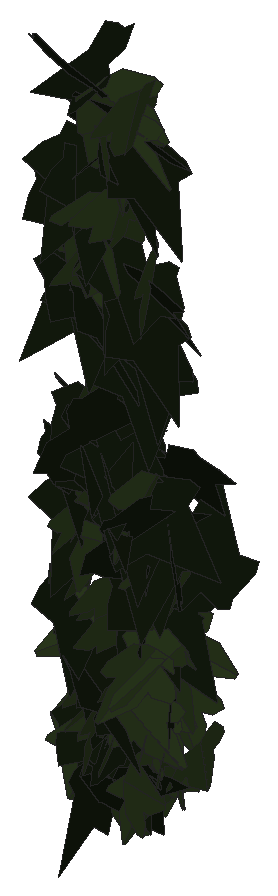
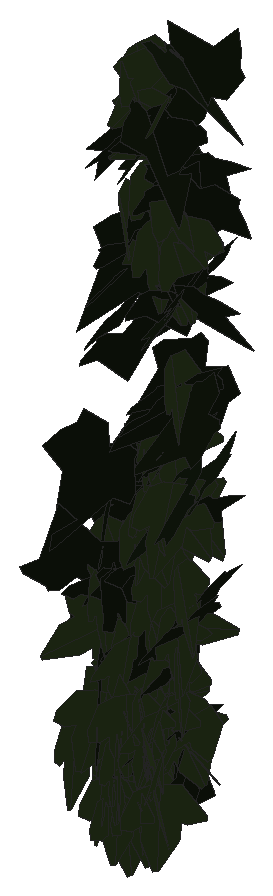
# SketchUp Ruby script. Lengths in inches.
U = 1.inch
M = Sketchup.active_model
def pt(a) = Geom::Point3d.new(a.map { |v| v * U })
def face(e, loops, mat)
  f = e.add_face(loops[0].map { |a| pt(a) })
  loops[1..].each { |l| e.add_face(l.map { |a| pt(a) }).erase! }
  f.material = f.back_material = mat if mat
  f
end
# faces: each face lists its corners as indices into pts; further lists are holes
def faces(e, pts, list, mat = nil) = list.each { |f| face(e, (f[0].is_a?(Array) ? f : [f]).map { |l| l.map { |i| pts[i] } }, mat) }
# xy, xz, yz: faces in a plane at the given z, y or x. An outline is a flat list of corners, or four numbers for a rectangle; further outlines are holes
def ring(l) = l.size == 4 ? [[l[0], l[1]], [l[2], l[1]], [l[2], l[3]], [l[0], l[3]]] : l.each_slice(2).to_a
def flat(e, list, mat, &to3) = list.each { |f| face(e, (f[0].is_a?(Array) ? f : [f]).map { |l| ring(l).map { |u, v| to3.(u, v) } }, mat) }
def xy(e, z, list, mat = nil) = flat(e, list, mat) { |x, y| [x, y, z] }
def xz(e, y, list, mat = nil) = flat(e, list, mat) { |x, z| [x, y, z] }
def yz(e, x, list, mat = nil) = flat(e, list, mat) { |y, z| [x, y, z] }
def lines(e, pts, list) = list.each { |a, b| e.add_line(pt(pts[a]), pt(pts[b])) }
# prism: a flat outline (further loops are holes) pulled along v
def prism(e, loops, v, mat = nil)
  f = face(e, loops, mat); d = Geom::Vector3d.new(v.map { |x| x * U })
  f.pushpull(f.normal.samedirection?(d) ? d.length : -d.length)
end
def box(e, o, s, mat = nil) = prism(e, [[o, [o[0] + s[0], o[1], o[2]], [o[0] + s[0], o[1] + s[1], o[2]], [o[0], o[1] + s[1], o[2]]]], [0, 0, s[2]], mat)
def at(x, y, z, deg = 0) = Geom::Transformation.translation(pt([x, y, z])) * Geom::Transformation.rotation(ORIGIN, Z_AXIS, deg.degrees)
def axes(o, x, y, z) = Geom::Transformation.new([*x, 0, *y, 0, *z, 0, *pt(o).to_a, 1])
def part(name) = M.definitions.add(name)
# library, detail: a bought-in or finely detailed component or shape, given as its bounding box
def library(name, o, s) = part(name).tap { |d| box(d.entities, o, s) }
def detail(e, o, s) = box(e.add_group.entities, o, s)
def put(e, d, t, mat = nil) = e.add_instance(d, t).tap { |i| i.material = mat if mat }
def group(e, t, mat = nil) = e.add_group.tap { |g| g.transformation = t; g.material = mat if mat }.entities
root = M.entities
M.materials.add("efeu1").color = [18, 25, 13]
M.materials.add("efeu2").color = [43, 57, 29]
c1 = part("ivyleaf_10")
p = [[0,0.5,-0.03],[-0.0625,2.02,-0.43],[-0.19,2.01,-0.46],[-0.54,1.05,-0.29],[-0.52,0.625,-0.18],[-0.83,0.76,-0.28],
  [-1.16,0.64,-0.33],[-1.15,0.33,-0.24],[-0.77,-0.39,0.02],[-0.3,-0.51,0.16],[0.04,-0.48,0.23],[-0.02,2.01,-0.4375],
  [-0.06,2.01,-0.43],[0.04,-0.49,0.23],[0.67,-0.49,0.14],[1.38,0.36,-0.2],[1.375,0.51,-0.24],[0.81,0.65,-0.19],
  [0.62,0.59,-0.15],[0.6,1.09,-0.28],[0.5,1.23,-0.31]]
faces(c1.entities,p,[[0,1,2,3,4,5,6,7,8,9,10],[11,12,0,13,14,15,16,17,18,19,20]],"efeu2")
c2 = part("ivyleaf_9")
p = [[1.54,2.16,1.25],[1.36,2.04,1.19],[-0.21,0.99,0.68],[-0.71,1.11,0.82],[-0.85,0.86,0.67],[-0.8,0.17,0.21],
  [-0.9,-0.01,0.1],[-0.67,-0.16,-0.02],[-0.08,-0.08,-0.05],[-0.03,-0.6,-0.4],[0.65,-0.88,-0.66],[0.83,-0.6,-0.49],
  [1.29,-0.42,-0.43],[1.8125,-0.07,-0.26],[1.21,0.44,0.15]]
faces(c2.entities,p,[[0,1,2,3,4,5,6,7,8,9,10,11,12,13,14]],"efeu1")
put(root,c1,axes([522.9,136.05,189.07],[0.22801,-0.734,-0.06651],[0.0034,0.07067,-0.76822],[0.737,0.22676,0.02413]))
put(root,c1,axes([522.96,136.78,184.16],[-0.49209,-0.52091,-0.02258],[0.01497,0.01693,-0.71659],[0.52118,-0.49232,-0.00074]))
put(root,c1,axes([522.77,137.04,185.41],[-0.32393,0.59208,-0.24043],[0.0853,-0.22708,-0.67414],[-0.63332,-0.33342,0.03218]))
put(root,c2,axes([523.13,135.86,195.8],[-0.757,-0.21652,-0.02581],[0.04509,-0.06421,-0.78386],[0.21334,-0.75471,0.07409]))
put(root,c1,axes([523.02,136.19,190.91],[-0.05988,-0.65964,0.38728],[-0.03191,-0.38597,-0.66234],[0.76426,-0.0678,0.00268]))
put(root,c1,axes([522.95,136.44,191.18],[-0.30759,-0.67798,-0.25733],[0.10884,0.2332,-0.74449],[0.71696,-0.32627,0.00262]))
put(root,c2,axes([522.56,135.78,191.38],[0.20078,-0.66191,0.37994],[0.12172,-0.36006,-0.69161],[0.75343,0.23456,0.01048]))
put(root,c2,axes([522.63,136.3125,191.39],[0.64613,-0.3981,-0.21204],[-0.14567,0.16642,-0.75631],[0.42688,0.65935,0.06287]))
put(root,c1,axes([523.03,135.97,187.07],[0.24664,-0.66818,-0.19615],[0.0004,0.20823,-0.70881],[0.69637,0.23653,0.06988]))
put(root,c2,axes([522.63,135.7,193.04],[0.73634,-0.23569,-0.03729],[-0.00848,0.09504,-0.76813],[0.23847,0.73113,0.08783]))
put(root,c1,axes([523.1,136.68,184.44],[0.35464,-0.63594,0.00442],[0.0179,0.00492,-0.72791],[0.6357,0.35463,0.01803]))
put(root,c1,axes([523.07,136.9,186.02],[-0.08547,0.70253,0.12456],[-0.06698,0.117,-0.70583],[-0.71034,-0.09557,0.05157]))
put(root,c1,axes([523.1875,135.875,187.9375],[-0.04746,-0.73603,-0.09381],[0.00368,0.09377,-0.73755],[0.74198,-0.04754,-0.00235]))
put(root,c2,axes([523.09,135.9,190.53],[-0.33698,-0.68499,0.15608],[-0.00786,-0.16943,-0.7605],[0.70251,-0.33048,0.06637]))
put(root,c1,axes([523.17,135.43,190.47],[0.11386,-0.65451,0.3887],[0.05706,-0.38458,-0.66429],[0.75908,0.12709,-0.00837]))
put(root,c1,axes([523.4375,135.84,187.73],[-0.20803,-0.01437,0.71782],[-0.25945,-0.69533,-0.08911],[0.66944,-0.27395,0.18853]))
put(root,c2,axes([523.71,135.47,201.09],[-0.57918,0.55506,0.11718],[-0.1882,-0.03002,-0.78801],[-0.53517,-0.59015,0.1503]))
put(root,c1,axes([523.27,135.73,185.28],[-0.25132,-0.6333,0.30957],[0.01622,-0.33376,-0.66963],[0.70472,-0.21816,0.12581]))
put(root,c1,axes([523.22,136.83,185.88],[0.32399,-0.64747,-0.0028],[-0.00193,0.00217,-0.72401],[0.64747,0.324,-0.00076]))
put(root,c2,axes([522.89,136.12,188.1],[0.15445,-0.74118,-0.1195],[0.00318,0.12265,-0.75659],[0.75074,0.15197,0.02779]))
put(root,c2,axes([522.97,135.53,188.37],[0.02585,-0.73587,0.19095],[0.00164,-0.191,-0.73631],[0.76024,0.02544,-0.00491]))
put(root,c2,axes([522.66,135.49,200.63],[0.06907,-0.43212,0.67428],[0.52997,-0.48274,-0.36366],[0.60043,0.4758,0.24342]))
put(root,c2,axes([523,135.375,198.11],[-0.46098,-0.32625,-0.55242],[0.45068,0.31946,-0.56475],[0.45661,-0.64468,-0.0003]))
put(root,c1,axes([523.68,136.33,185.69],[0.07687,0.06986,-0.77003],[-0.49935,0.59529,0.00416],[0.59032,0.49446,0.10379]))
put(root,c1,axes([523.33,136.76,186.3],[0.12341,-0.7267,-0.07436],[0.0026,0.07586,-0.73695],[0.73049,0.1225,0.01519]))
put(root,c1,axes([522.91,135.68,185.77],[-0.33343,-0.28876,-0.59565],[0.58188,0.19011,-0.41788],[0.31559,-0.65561,0.14117]))
put(root,c2,axes([522.98,135.27,196.19],[0.38907,-0.64319,-0.29751],[-0.10723,0.28206,-0.75002],[0.7005,0.40042,0.05043]))
put(root,c2,axes([523.37,135.59,198.68],[-0.58239,-0.55228,-0.01289],[0.06239,-0.04714,-0.7989],[0.5489,-0.58062,0.07713]))
put(root,c1,axes([523.43,135.46,196.64],[-0.0365,-0.80712,0.01247],[-0.00146,-0.01242,-0.80794],[0.80721,-0.03651,-0.0009]))
put(root,c1,axes([523.4,135.66,193.71],[0.1842,-0.76303,-0.14466],[-0.00515,0.14747,-0.78441],[0.77661,0.18196,0.02911]))
put(root,c1,axes([523.45,135.8,186.72],[-0.15579,-0.72339,-0.16286],[0.01642,0.16301,-0.73976],[0.74131,-0.15564,-0.01784]))
put(root,c1,axes([523.37,136.22,186],[-0.35998,0.64639,0.04082],[-0.02206,0.03443,-0.73987],[-0.6473,-0.36065,0.00252]))
put(root,c1,axes([523.6,136.64,186.07],[0.26618,-0.48712,-0.4683],[-0.23308,0.40624,-0.55505],[0.63424,0.35373,-0.00744]))
put(root,c1,axes([523.56,136.32,185.92],[-0.55159,-0.45539,0.08035],[-0.05933,-0.05433,-0.71527],[0.4586,-0.55476,0.0041]))
put(root,c1,axes([523.57,136.13,186.14],[-0.06765,0.20523,-0.7114],[-0.26545,-0.6736,-0.16908],[-0.69119,0.2386,0.13456]))
put(root,c2,axes([523.28,135.75,184.16],[-0.01714,0.05335,-0.77052],[0.53869,-0.55149,-0.05017],[-0.55351,-0.53838,-0.02497]))
put(root,c2,axes([524.08,135.57,185.51],[-0.53478,0.459,0.33561],[-0.27812,0.1907,-0.70398],[-0.49595,-0.60187,0.03289]))
put(root,c1,axes([523.67,135.36,197.8125],[-0.15648,-0.72443,0.28072],[-0.06424,-0.27332,-0.74112],[0.77426,-0.16909,-0.00476]))
put(root,c1,axes([523.63,136.61,183.95],[-0.23517,-0.68863,0.0359],[-0.01364,-0.03328,-0.72767],[0.68943,-0.23555,-0.00215]))
put(root,c1,axes([523.625,135.11,196.96],[0.74213,-0.09213,-0.2567],[-0.21813,0.24621,-0.71899],[0.16371,0.74567,0.20568]))
put(root,c1,axes([523.61,137.08,186.22],[-0.50702,-0.51288,0.04323],[0.05989,-0.11907,-0.71008],[0.5112,-0.49474,0.12607]))
put(root,c2,axes([523.92,135.42,199.31],[-0.11065,0.78295,0.17358],[-0.15154,0.15166,-0.78065],[-0.78751,-0.13919,0.12583]))
put(root,c2,axes([523.44,135.85,195.78],[-0.26829,-0.73879,-0.08469],[0.03351,0.07793,-0.78599],[0.74288,-0.27033,0.00487]))
put(root,c1,axes([523.53,136.23,185.625],[0.28656,-0.6458,0.24341],[0.11779,-0.21392,-0.70625],[0.68002,0.3092,0.01976]))
put(root,c2,axes([523.42,135.72,198.32],[-0.16863,-0.77685,-0.00116],[0.00022,0.00114,-0.79494],[0.77685,-0.16863,-0.00003]))
put(root,c2,axes([523.24,135.81,185.69],[0.06876,-0.62459,-0.43477],[0.14237,0.43939,-0.60871],[0.74757,-0.02623,0.15591]))
put(root,c2,axes([523.47,135.82,186.45],[0.27047,-0.39164,-0.60337],[-0.31122,0.51745,-0.47538],[0.64852,0.41165,0.02351]))
put(root,c2,axes([523.36,136.32,185.1],[0.1117,-0.69257,-0.31477],[-0.01986,0.31538,-0.70096],[0.76048,0.10996,0.02793]))
put(root,c1,axes([523.55,135.74,185.93],[-0.25835,-0.51949,-0.50038],[0.2821,0.4164,-0.57795],[0.66383,-0.37912,0.05087]))
put(root,c1,axes([523.79,136.9,183.8],[-0.41742,-0.57764,0.05217],[-0.02988,-0.04278,-0.71267],[0.57922,-0.41849,0.00083]))
put(root,c1,axes([523.8,135.3125,192.02],[-0.35065,-0.6925,0.04126],[-0.01359,-0.03937,-0.7762],[0.6936,-0.35087,0.00566]))
put(root,c1,axes([523.84,137.13,184.16],[-0.70847,-0.08584,0.09967],[-0.09751,-0.0237,-0.71355],[0.08828,-0.71505,0.01169]))
put(root,c1,axes([523.78,135.94,185.43],[0.20561,-0.68349,-0.24067],[-0.03084,0.24169,-0.71274],[0.72397,0.20441,0.03799]))
put(root,c1,axes([523.72,135.49,186.33],[0.34411,-0.78039,0.13756],[0.03769,-0.13369,-0.85267],[0.79153,0.34563,-0.0192]))
put(root,c1,axes([523.8125,136.21,190.25],[-0.19559,-0.69304,0.2364],[-0.00556,-0.24328,-0.71779],[0.73223,-0.18697,0.05769]))
put(root,c1,axes([523.8125,135.64,188.97],[-0.20364,-0.71541,-0.11352],[0.0147,0.11382,-0.74364],[0.72421,-0.20347,-0.01683]))
put(root,c2,axes([523.43,135.47,192],[0.17427,-0.73716,-0.12165],[-0.00006,0.1249,-0.75695],[0.74713,0.17195,0.02831]))
put(root,c1,axes([523.79,135.76,196.9],[-0.12095,-0.78256,-0.05289],[0.05406,0.04507,-0.79048],[0.78248,-0.12407,0.04644]))
put(root,c2,axes([523.47,135.61,192.51],[0.10452,-0.68012,0.38885],[0.02721,-0.38891,-0.68753],[0.78296,0.10431,-0.02802]))
put(root,c1,axes([523.85,135.64,188.11],[-0.19631,-0.71421,-0.12632],[0.0204,0.12538,-0.74057],[0.725,-0.19691,-0.01336]))
put(root,c1,axes([523.86,136.84,185.21],[0.19542,-0.65065,-0.2868],[-0.00363,0.29652,-0.67517],[0.71105,0.18033,0.07538]))
put(root,c1,axes([523.84,135.65,196.39],[0.76413,0.12089,-0.18392],[-0.19494,0.06325,-0.76833],[-0.10218,0.7834,0.09042]))
put(root,c2,axes([523.4,135.62,195.45],[0.4101,-0.68862,0.00741],[0.01178,-0.00161,-0.80143],[0.68856,0.41016,0.0093]))
put(root,c1,axes([523.99,136.93,185.54],[-0.51825,0.43433,0.25704],[-0.22222,0.13441,-0.67517],[-0.45313,-0.56266,0.03713]))
put(root,c1,axes([523.89,136.92,185.07],[-0.00775,-0.69357,-0.19751],[0.03023,0.19703,-0.69308],[0.72051,-0.01573,0.02696]))
put(root,c2,axes([523.79,134.35,193.11],[-0.03509,0.18184,-0.90896],[-0.28055,0.86486,0.18385],[0.88349,0.28186,0.02229]))
put(root,c1,axes([523.9,135.47,191.43],[0.12756,-0.69093,0.30369],[0.03973,-0.30143,-0.70246],[0.75368,0.13283,-0.01437]))
put(root,c2,axes([523.56,135.39,193.24],[0.04027,-0.7129,-0.31599],[0.07927,0.31852,-0.70849],[0.77576,0.00446,0.0888]))
put(root,c2,axes([523.3,135.45,199.8],[0.72758,-0.07712,0.3361],[0.33828,0.00739,-0.73062],[0.0669,0.80143,0.03908]))
put(root,c2,axes([523.53,135.15,187.03],[0.5405,-0.61004,-0.03095],[-0.01952,0.02405,-0.81504],[0.61052,0.54085,0.00134]))
put(root,c2,axes([523.7,135.94,186.41],[0.3495,-0.65413,-0.27341],[-0.13189,0.23952,-0.74164],[0.6966,0.37354,-0.00324]))
put(root,c1,axes([523.86,134.84,190.4],[-0.02384,-0.46359,-0.65844],[0.27785,0.61354,-0.44204],[0.75582,-0.24017,0.14173]))
put(root,c1,axes([524.1,136.34,186.09],[0.39533,0.47162,-0.37486],[-0.28138,-0.25191,-0.61368],[-0.5327,0.48306,0.04596]))
put(root,c1,axes([524.0625,135.8,190.39],[0.07111,-0.69905,-0.33591],[0.02776,0.3394,-0.70043],[0.77507,0.05198,0.05591]))
put(root,c2,axes([523.95,135.53,184.45],[0.59512,0.55736,-0.0919],[-0.07356,-0.05589,-0.81531],[-0.56007,0.59957,0.00943]))
put(root,c1,axes([523.99,136.6,187.39],[-0.02202,0.72956,0.00263],[-0.04034,0.00141,-0.72878],[-0.72845,-0.02213,0.04028]))
put(root,c1,axes([523.99,136.94,184.36],[0.66223,-0.30568,0.00153],[0.01016,0.01837,-0.72908],[0.30551,0.66198,0.02094]))
put(root,c1,axes([524.16,135.39,198.1],[-0.17823,-0.78364,0.13694],[0.00018,-0.14038,-0.80306],[0.79551,-0.17554,0.03087]))
put(root,c2,axes([523.86,135.8,187.31],[-0.02691,-0.58734,-0.53182],[-0.01278,0.53238,-0.58731],[0.79224,-0.01136,-0.02754]))
put(root,c2,axes([523.9,135.95,192.74],[-0.04061,-0.7675,0.06321],[-0.01956,-0.06225,-0.76841],[0.76985,-0.04207,-0.01619]))
put(root,c1,axes([523.97,136.82,185.55],[-0.65913,0.00623,-0.29854],[0.28887,-0.16994,-0.64132],[-0.07563,-0.70334,0.15231]))
put(root,c1,axes([523.66,136.45,185.15],[-0.16761,0.08875,-0.75291],[0.56596,-0.4984,-0.18474],[-0.50442,-0.5887,0.0429]))
put(root,c1,axes([524.0625,136.63,186.05],[0.49277,-0.51482,0.20548],[0.13456,-0.15562,-0.71257],[0.53773,0.51071,-0.00999]))
put(root,c1,axes([524.21,135.52,191.43],[0.24534,-0.68859,-0.20788],[0.00591,0.22156,-0.72693],[0.71926,0.23306,0.07688]))
put(root,c1,axes([524.11,135.12,199.6875],[-0.28703,0.74356,-0.07563],[0.03497,-0.06757,-0.79699],[-0.74657,-0.28903,-0.00825]))
put(root,c2,axes([523.83,135.5,191.48],[0.18821,-0.71251,0.29751],[0.13596,-0.27085,-0.73468],[0.76006,0.22488,0.05775]))
put(root,c1,axes([523.99,135.27,200.57],[-0.52828,-0.33645,-0.52555],[0.4696,0.23911,-0.62512],[0.41094,-0.70577,0.03875]))
put(root,c1,axes([523.92,135.48,199.61],[-0.58605,-0.11385,-0.54676],[0.55059,0.01498,-0.59328],[0.09355,-0.80136,0.06659]))
put(root,c2,axes([524.16,135.39,192.41],[-0.14578,-0.75355,-0.06555],[0.00669,0.06547,-0.7675],[0.75637,-0.14581,-0.00585]))
put(root,c1,axes([524.38,136.95,184.45],[0.55307,-0.42964,-0.20857],[0.01207,0.33159,-0.65106],[0.47743,0.48933,0.25806]))
put(root,c1,axes([524.53,136.71,186.42],[0.64691,-0.19465,-0.31456],[-0.21958,0.30792,-0.6421],[0.2977,0.65009,0.20995]))
put(root,c1,axes([524.52,136.02,184.45],[-0.15388,-0.65037,0.30454],[-0.02405,-0.30661,-0.66695],[0.71774,-0.14971,0.04294]))
put(root,c1,axes([524.39,136.98,185.97],[-0.648,-0.29707,-0.16107],[0.17859,-0.00533,-0.70864],[0.28688,-0.6677,0.07732]))
put(root,c2,axes([524.08,135.62,199.18],[0.37764,-0.70336,0.07002],[0.01846,-0.06955,-0.79815],[0.70659,0.37773,-0.01657]))
put(root,c2,axes([524.83,136.31,186.6],[0.10069,-0.05214,-0.7918],[-0.72623,0.31559,-0.11314],[0.31977,0.73313,-0.00761]))
put(root,c1,axes([524.61,135.31,200.58],[-0.03303,-0.81514,0.01147],[-0.00086,-0.01145,-0.81581],[0.81522,-0.03304,-0.0004]))
put(root,c1,axes([524.7,135.93,187.56],[-0.7074,-0.16324,0.07957],[-0.07588,-0.02501,-0.72595],[0.16498,-0.71142,0.00727]))
put(root,c2,axes([524.41,135.89,191.09],[-0.16433,-0.74586,-0.09981],[0.02372,0.09697,-0.76374],[0.75213,-0.16602,0.00228]))
put(root,c1,axes([524.72,136.24,185.39],[0.25641,-0.5036,-0.45479],[-0.1237,0.44334,-0.56066],[0.66719,0.27574,0.07083]))
put(root,c2,axes([524.3125,136.1,188.94],[0.14814,-0.71982,-0.27685],[-0.03428,0.27549,-0.73461],[0.77046,0.15066,0.02055]))
put(root,c1,axes([524.75,135.18,184.74],[-0.16191,0.46259,0.62237],[-0.27851,0.55868,-0.48771],[-0.72372,-0.31849,0.04845]))
put(root,c2,axes([524.57,135.69,196.5],[-0.37073,-0.70487,0.06755],[0.00914,-0.081,-0.79511],[0.70804,-0.36803,0.04563]))
put(root,c2,axes([524.54,136.16,187.97],[-0.00741,0.41853,0.67624],[-0.20147,-0.6552,0.4033],[0.76934,-0.16755,0.11213]))
put(root,c1,axes([524.78,136.39,188.54],[0.09712,-0.72908,-0.13783],[0.00006,0.13901,-0.7353],[0.74199,0.09542,0.0181]))
put(root,c2,axes([524.44,135.45,196.4],[0.8144,0.01201,-0.13431],[-0.13439,0.0046,-0.81446],[-0.01111,0.82539,0.0065]))
put(root,c1,axes([524.92,135.26,187.61],[0.28401,0.5147,-0.46604],[-0.38746,-0.30035,-0.56783],[-0.57618,0.45568,0.15212]))
put(root,c2,axes([524.59,134.58,190.73],[-0.03955,0.4193,-0.70981],[-0.09616,0.70343,0.42089],[0.81878,0.10286,0.01514]))
put(root,c1,axes([524.76,135.45,191.52],[0.05127,-0.63069,0.43616],[0.11869,-0.42534,-0.62899],[0.75758,0.10932,0.06903]))
put(root,c1,axes([524.53,135.51,186.22],[-0.52808,-0.2354,-0.43997],[0.45095,0.04907,-0.56752],[0.21359,-0.68558,0.11044]))
put(root,c2,axes([524.63,136.47,191.84],[0.75552,0.27204,-0.16937],[-0.16236,-0.049,-0.80296],[-0.27628,0.77272,0.00871]))
put(root,c2,axes([524.62,135.87,194.375],[-0.13214,-0.75978,-0.12015],[0.0107,0.12009,-0.77112],[0.76914,-0.1322,-0.00992]))
put(root,c2,axes([524.66,135.87,190.44],[-0.30335,-0.60901,-0.34469],[0.15769,0.30652,-0.68037],[0.68179,-0.34187,0.004]))
put(root,c2,axes([524.78,135.79,190.43],[-0.43128,-0.60944,-0.25471],[0.12634,0.22247,-0.74622],[0.64833,-0.44876,-0.02402]))
put(root,c1,axes([524.95,135.91,189.55],[-0.14577,-0.71295,0.21921],[0.00827,-0.22488,-0.72592],[0.74584,-0.13685,0.05089]))
put(root,c2,axes([524.52,135.73,199.16],[0.21063,-0.73632,-0.18532],[0.03768,0.20222,-0.76064],[0.75835,0.19447,0.08926]))
put(root,c1,axes([525.08,135.76,187.64],[-0.22757,-0.3458,0.63338],[-0.11674,-0.63774,-0.39012],[0.71212,-0.21505,0.13846]))
put(root,c2,axes([524.63,136.03,188.48],[0.0192,-0.51694,-0.59518],[0.11317,0.591,-0.50965],[0.78017,-0.073,0.08858]))
put(root,c1,axes([525.09,136.85,185.01],[-0.05513,-0.67514,-0.28163],[0.00202,0.28228,-0.67711],[0.73152,-0.05166,-0.01935]))
put(root,c2,axes([524.67,135.4375,191.21],[0.08554,-0.38612,-0.69976],[0.15494,0.69842,-0.36644],[0.78406,-0.0959,0.14876]))
put(root,c2,axes([524.77,135.83,194.9],[0.10391,-0.76514,0.1623],[0.01062,-0.16233,-0.77209],[0.78209,0.10386,-0.01108]))
put(root,c2,axes([525.27,135.91,189.3],[0.13317,-0.43472,0.65491],[-0.05813,0.65698,0.44792],[-0.78391,-0.12257,0.07804]))
put(root,c1,axes([524.99,135.375,196.97],[0.39008,-0.68075,0.16164],[0.15858,-0.09423,-0.77954],[0.68147,0.4116,0.08887]))
put(root,c2,axes([525.17,136.78,188.86],[-0.59703,-0.25849,0.507],[0.4703,0.18966,0.65051],[-0.32045,0.75995,0.0101]))
put(root,c2,axes([524.81,135.375,195.65],[0.20373,-0.75786,-0.1581],[0.02828,0.17065,-0.78162],[0.77365,0.19333,0.0702]))
put(root,c1,axes([524.75,136.37,187.59],[0.26226,0.22393,0.65302],[0.39964,0.52036,-0.33894],[-0.56291,0.47376,0.06361]))
